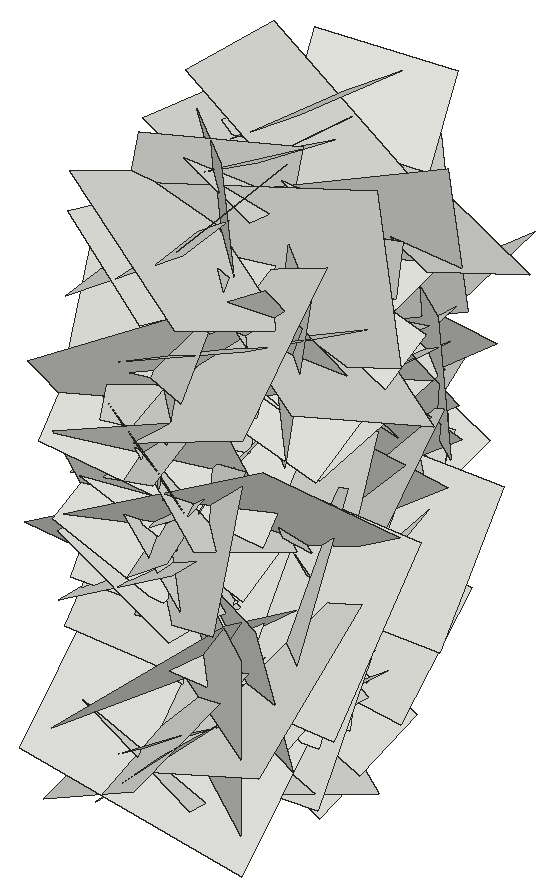
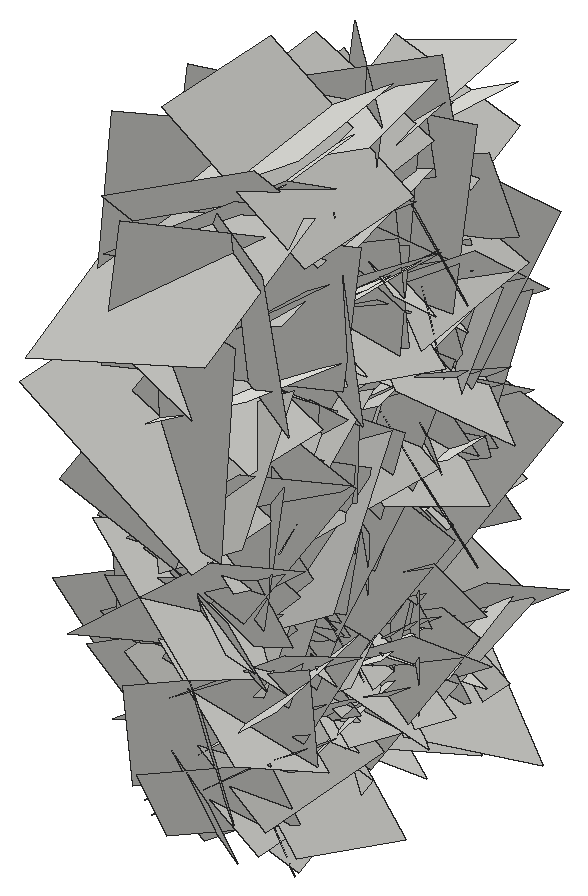
# SketchUp Ruby script. Lengths in inches.
U = 1.inch
M = Sketchup.active_model
def pt(a) = Geom::Point3d.new(a.map { |v| v * U })
def face(e, loops, mat)
  f = e.add_face(loops[0].map { |a| pt(a) })
  loops[1..].each { |l| e.add_face(l.map { |a| pt(a) }).erase! }
  f.material = f.back_material = mat if mat
  f
end
# faces: each face lists its corners as indices into pts; further lists are holes
def faces(e, pts, list, mat = nil) = list.each { |f| face(e, (f[0].is_a?(Array) ? f : [f]).map { |l| l.map { |i| pts[i] } }, mat) }
# xy, xz, yz: faces in a plane at the given z, y or x. An outline is a flat list of corners, or four numbers for a rectangle; further outlines are holes
def ring(l) = l.size == 4 ? [[l[0], l[1]], [l[2], l[1]], [l[2], l[3]], [l[0], l[3]]] : l.each_slice(2).to_a
def flat(e, list, mat, &to3) = list.each { |f| face(e, (f[0].is_a?(Array) ? f : [f]).map { |l| ring(l).map { |u, v| to3.(u, v) } }, mat) }
def xy(e, z, list, mat = nil) = flat(e, list, mat) { |x, y| [x, y, z] }
def xz(e, y, list, mat = nil) = flat(e, list, mat) { |x, z| [x, y, z] }
def yz(e, x, list, mat = nil) = flat(e, list, mat) { |y, z| [x, y, z] }
def lines(e, pts, list) = list.each { |a, b| e.add_line(pt(pts[a]), pt(pts[b])) }
# prism: a flat outline (further loops are holes) pulled along v
def prism(e, loops, v, mat = nil)
  f = face(e, loops, mat); d = Geom::Vector3d.new(v.map { |x| x * U })
  f.pushpull(f.normal.samedirection?(d) ? d.length : -d.length)
end
def box(e, o, s, mat = nil) = prism(e, [[o, [o[0] + s[0], o[1], o[2]], [o[0] + s[0], o[1] + s[1], o[2]], [o[0], o[1] + s[1], o[2]]]], [0, 0, s[2]], mat)
def at(x, y, z, deg = 0) = Geom::Transformation.translation(pt([x, y, z])) * Geom::Transformation.rotation(ORIGIN, Z_AXIS, deg.degrees)
def axes(o, x, y, z) = Geom::Transformation.new([*x, 0, *y, 0, *z, 0, *pt(o).to_a, 1])
def part(name) = M.definitions.add(name)
# library, detail: a bought-in or finely detailed component or shape, given as its bounding box
def library(name, o, s) = part(name).tap { |d| box(d.entities, o, s) }
def detail(e, o, s) = box(e.add_group.entities, o, s)
def put(e, d, t, mat = nil) = e.add_instance(d, t).tap { |i| i.material = mat if mat }
def group(e, t, mat = nil) = e.add_group.tap { |g| g.transformation = t; g.material = mat if mat }.entities
root = M.entities
c1 = part("Component\#6")
p = [[0.01,0,0],[0,3.24,4.54],[4.32,3.24,4.54],[4.33,0,0]]
faces(c1.entities,p,[[0,1,2,3]])
put(root,c1,axes([34.14,144.73,33.27],[-0.16555,-0.76551,-0.15352],[0.02389,-0.16091,0.77946],[0.82725,-0.14855,-0.05323]))
put(root,c1,axes([34.14,146.45,21.25],[-0.00375,0.2874,0.54008],[0.0654,0.5375,-0.28562],[0.64519,-0.05282,0.03209]))
put(root,c1,axes([34.14,136.92,29.78],[0.03864,0.57092,0.32429],[-0.05823,0.3263,-0.56829],[0.69355,-0.00442,-0.06578]))
put(root,c1,axes([34.14,144.18,33.46],[-0.08879,-0.56105,-0.39599],[0.0694,-0.40364,0.55803],[0.72461,-0.03009,-0.10197]))
put(root,c1,axes([38.11,149.17,29.19],[-0.22051,-0.77582,-0.34275],[0.07369,-0.36732,0.78924],[-0.89602,0.16072,0.14925]))
put(root,c1,axes([34.14,141.16,33.73],[0.01034,-0.20439,-0.70125],[-0.11317,-0.69418,0.20085],[0.76594,-0.09981,0.03914]))
put(root,c1,axes([34.14,145.72,37.21],[0.0202,-0.65006,0.07365],[-0.02062,0.07308,0.65011],[0.69316,0.02112,0.01719]))
put(root,c1,axes([34.14,146.3,23.53],[-0.0913,-0.50535,0.50896],[0.05568,0.5068,0.51209],[0.75823,-0.09807,0.02368]))
put(root,c1,axes([34.14,145.7,22.51],[-0.08358,0.19729,0.79599],[-0.0899,0.79341,-0.20506],[0.86462,0.10156,0.05562]))
put(root,c1,axes([38.11,145.12,23.07],[0.0526,-0.82286,-0.58821],[-0.0059,-0.58914,0.82367],[-1.07215,-0.03713,-0.03339]))
put(root,c1,axes([34.14,147.44,21.48],[0.11936,-0.32986,-0.48912],[-0.02265,-0.49991,0.33221],[0.62494,0.04489,0.10546]))
put(root,c1,axes([38.11,137.68,27.62],[-0.00267,0.49736,0.77514],[-0.05686,0.77375,-0.49665],[-0.97459,-0.04651,0.02685]))
put(root,c1,axes([38.11,136.3,32.46],[0.17238,0.91042,0.71253],[0.07022,0.71102,-0.92361],[-1.22345,0.16908,0.04738]))
put(root,c1,axes([34.14,137.77,24.11],[-0.1419,0.78136,-0.16109],[0.04598,-0.15597,-0.79258],[0.84441,0.13979,0.01609]))
put(root,c1,axes([34.14,143.53,22.21],[-0.15224,-0.84766,-0.36991],[-0.10957,-0.35729,0.85887],[0.97421,-0.17265,0.03879]))
put(root,c1,axes([38.11,135.48,23.28],[0.21581,1.04519,0.5846],[0.09636,0.57779,-1.06467],[-1.26577,0.22219,0.01862]))
put(root,c1,axes([34.14,145.6,27.28],[0.00806,0.29423,-0.56577],[0.12293,-0.55701,-0.28812],[0.6647,0.09945,0.06014]))
put(root,c1,axes([38.11,141.63,23.18],[0.01995,1.00092,0.30572],[0.13829,0.30114,-0.99396],[-1.10071,0.05598,-0.11933]))
put(root,c1,axes([38.11,145.42,24.52],[0.2647,-0.88765,0.75819],[0.01358,0.77738,0.90589],[-1.23735,-0.18136,0.17214]))
put(root,c1,axes([34.14,144.6,22.65],[-0.17478,-0.82558,-0.09028],[0.09417,-0.10904,0.83495],[0.87528,-0.15312,-0.10786]))
put(root,c1,axes([38.11,142.67,41.25],[0.05619,0.9574,-0.08237],[-0.00834,-0.08206,-0.95886],[-1.01856,0.05349,0.00331]))
put(root,c1,axes([38.11,148.52,32.35],[-0.08011,-0.79067,-0.06214],[-0.07476,-0.05548,0.79163],[-0.83736,0.0806,-0.06473]))
put(root,c1,axes([34.14,140.84,40.56],[-0.05261,0.712,-0.12967],[0.10362,-0.12219,-0.70833],[0.7601,0.06594,0.08758]))
put(root,c1,axes([34.14,143.38,25.93],[-0.00088,-0.66729,0.07011],[0.1194,0.06898,0.65784],[0.70113,-0.01259,-0.11194]))
put(root,c1,axes([34.14,144.05,31.85],[-0.11078,0.17753,-0.74918],[0.12323,-0.74375,-0.19246],[0.80677,0.13798,-0.07348]))
put(root,c1,axes([38.11,138.53,29.67],[-0.03677,-0.4198,0.69058],[-0.10131,0.68849,0.41374],[-0.85065,-0.06385,-0.07912]))
put(root,c1,axes([38.11,150.98,27.43],[-0.11329,-0.77541,-0.3635],[0.07754,-0.37325,0.77469],[-0.90445,0.06513,0.11195]))
put(root,c1,axes([38.11,149.13,24.11],[0.03147,-0.85153,-0.39996],[0.02133,-0.3995,0.85202],[-0.997,-0.03542,0.00561]))
put(root,c1,axes([38.11,144.71,33.13],[0.16995,0.04512,1.05289],[0.00982,1.0649,-0.04705],[-1.11704,0.01623,0.15977]))
put(root,c1,axes([34.14,143.64,28.51],[0.01569,-0.00258,-0.72773],[0.02057,-0.72762,0.00297],[0.77112,0.01947,0.01473]))
put(root,c1,axes([38.11,137.85,30.84],[0.06669,0.91948,0.38333],[0.06841,0.37952,-0.92095],[-1.05374,0.08283,-0.03553]))
put(root,c1,axes([38.11,147.08,31.53],[0.0186,0.21399,-0.90436],[0.04027,-0.90393,-0.21315],[-0.98427,-0.03294,-0.02581]))
put(root,c1,axes([34.14,144.98,23.12],[0.11015,0.70988,0.06167],[-0.04855,0.06885,-0.71532],[0.75374,-0.09931,-0.05509]))
put(root,c1,axes([34.14,140.76,35.5625],[0.0095,0.80566,-0.00603],[-0.04784,-0.00552,-0.80445],[0.85268,-0.00929,-0.04507]))
put(root,c1,axes([34.14,146.7,34.04],[-0.22474,0.77203,-0.6543],[-0.03576,-0.67353,-0.78378],[1.07212,0.13937,-0.1633]))
put(root,c1,axes([38.11,141.61,27.46],[0.15544,0.8369,-0.58263],[0.03072,-0.5918,-0.84279],[-1.08048,0.10358,-0.10778]))
put(root,c1,axes([38.11,145.6875,25.3],[0.21495,-0.77208,-0.77151],[0.06755,-0.77499,0.79232],[-1.15499,-0.18901,-0.09724]))
put(root,c1,axes([38.11,147.86,21.63],[0.08807,-1.00346,0.13322],[0.11481,0.14172,0.99989],[-1.06685,-0.06759,0.1186]))
put(root,c1,axes([34.14,139.84,37.375],[0.13047,0.02824,0.77],[-0.11824,0.77221,-0.01049],[0.80815,0.10842,-0.12584]))
put(root,c1,axes([38.11,144.76,23.61],[-0.10873,-0.7568,0.02149],[0.01122,0.02025,0.76368],[-0.80245,0.10283,0.00777]))
put(root,c1,axes([34.14,149.44,28.46],[-0.01637,-0.35652,-0.61871],[0.18604,-0.60176,0.34238],[0.7337,0.14463,-0.10062]))
put(root,c1,axes([34.14,137.14,29.31],[0.00249,0.75761,-0.01469],[0.08098,-0.01485,-0.75375],[0.79913,-0.00085,0.07643]))
put(root,c1,axes([34.14,137.53,34.5],[-0.08019,0.3809,0.76753],[0.04804,0.77121,-0.37826],[0.90698,-0.00717,0.08789]))
put(root,c1,axes([38.11,139.47,36.72],[-0.15825,-0.66033,0.08813],[-0.02764,0.09604,0.67542],[-0.70562,0.14433,-0.04622]))
put(root,c1,axes([34.14,139.47,36.72],[0.15825,-0.66033,0.08813],[0.02764,0.09604,0.67542],[0.70562,0.14433,-0.04622]))
put(root,c1,axes([38.11,137.53,34.5],[0.08019,0.3809,0.76753],[-0.04804,0.77121,-0.37826],[-0.90698,-0.00717,0.08789]))
put(root,c1,axes([38.11,137.14,29.31],[-0.00249,0.75761,-0.01469],[-0.08098,-0.01485,-0.75375],[-0.79913,-0.00085,0.07643]))
put(root,c1,axes([38.11,149.44,28.46],[0.01637,-0.35652,-0.61871],[-0.18604,-0.60176,0.34238],[-0.7337,0.14463,-0.10062]))
put(root,c1,axes([34.14,144.76,23.61],[0.10873,-0.7568,0.02149],[-0.01122,0.02025,0.76368],[0.80245,0.10283,0.00777]))
put(root,c1,axes([38.11,139.84,37.375],[-0.13047,0.02824,0.77],[0.11824,0.77221,-0.01049],[-0.80815,0.10842,-0.12584]))
put(root,c1,axes([34.14,147.86,21.63],[-0.08807,-1.00346,0.13322],[-0.11481,0.14172,0.99989],[1.06685,-0.06759,0.1186]))
put(root,c1,axes([34.14,145.6875,25.3],[-0.21495,-0.77208,-0.77151],[-0.06755,-0.77499,0.79232],[1.15499,-0.18901,-0.09724]))
put(root,c1,axes([34.14,141.61,27.46],[-0.15544,0.8369,-0.58263],[-0.03072,-0.5918,-0.84279],[1.08048,0.10358,-0.10778]))
put(root,c1,axes([38.11,146.7,34.04],[0.22474,0.77203,-0.6543],[0.03576,-0.67353,-0.78378],[-1.07212,0.13937,-0.1633]))
put(root,c1,axes([38.11,140.76,35.5625],[-0.0095,0.80566,-0.00603],[0.04784,-0.00552,-0.80445],[-0.85268,-0.00929,-0.04507]))
put(root,c1,axes([38.11,144.98,23.12],[-0.11015,0.70988,0.06167],[0.04855,0.06885,-0.71532],[-0.75374,-0.09931,-0.05509]))
put(root,c1,axes([34.14,147.08,31.53],[-0.0186,0.21399,-0.90436],[-0.04027,-0.90393,-0.21315],[0.98427,-0.03294,-0.02581]))
put(root,c1,axes([34.14,137.85,30.84],[-0.06669,0.91948,0.38333],[-0.06841,0.37952,-0.92095],[1.05374,0.08283,-0.03553]))
put(root,c1,axes([38.11,143.64,28.51],[-0.01569,-0.00258,-0.72773],[-0.02057,-0.72762,0.00297],[-0.77112,0.01947,0.01473]))
put(root,c1,axes([34.14,144.71,33.13],[-0.16995,0.04512,1.05289],[-0.00982,1.0649,-0.04705],[1.11704,0.01623,0.15977]))
put(root,c1,axes([34.14,149.13,24.11],[-0.03147,-0.85153,-0.39996],[-0.02133,-0.3995,0.85202],[0.997,-0.03542,0.00561]))
put(root,c1,axes([34.14,150.98,27.43],[0.11329,-0.77541,-0.3635],[-0.07754,-0.37325,0.77469],[0.90445,0.06513,0.11195]))
put(root,c1,axes([34.14,138.53,29.67],[0.03677,-0.4198,0.69058],[0.10131,0.68849,0.41374],[0.85065,-0.06385,-0.07912]))
put(root,c1,axes([38.11,144.05,31.85],[0.11078,0.17753,-0.74918],[-0.12323,-0.74375,-0.19246],[-0.80677,0.13798,-0.07348]))
put(root,c1,axes([38.11,143.38,25.93],[0.00088,-0.66729,0.07011],[-0.1194,0.06898,0.65784],[-0.70113,-0.01259,-0.11194]))
put(root,c1,axes([38.11,140.84,40.56],[0.05261,0.712,-0.12967],[-0.10362,-0.12219,-0.70833],[-0.7601,0.06594,0.08758]))
put(root,c1,axes([34.14,148.52,32.35],[0.08011,-0.79067,-0.06214],[0.07476,-0.05548,0.79163],[0.83736,0.0806,-0.06473]))
put(root,c1,axes([34.14,142.67,41.25],[-0.05619,0.9574,-0.08237],[0.00834,-0.08206,-0.95886],[1.01856,0.05349,0.00331]))
put(root,c1,axes([38.11,144.6,22.65],[0.17478,-0.82558,-0.09028],[-0.09417,-0.10904,0.83495],[-0.87528,-0.15312,-0.10786]))
put(root,c1,axes([34.14,145.42,24.52],[-0.2647,-0.88765,0.75819],[-0.01358,0.77738,0.90589],[1.23735,-0.18136,0.17214]))
put(root,c1,axes([34.14,141.63,23.18],[-0.01995,1.00092,0.30572],[-0.13829,0.30114,-0.99396],[1.10071,0.05598,-0.11933]))
put(root,c1,axes([38.11,145.6,27.28],[-0.00806,0.29423,-0.56577],[-0.12293,-0.55701,-0.28812],[-0.6647,0.09945,0.06014]))
put(root,c1,axes([34.14,135.48,23.28],[-0.21581,1.04519,0.5846],[-0.09636,0.57779,-1.06467],[1.26577,0.22219,0.01862]))
put(root,c1,axes([38.11,143.53,22.21],[0.15224,-0.84766,-0.36991],[0.10957,-0.35729,0.85887],[-0.97421,-0.17265,0.03879]))
put(root,c1,axes([38.11,137.77,24.11],[0.1419,0.78136,-0.16109],[-0.04598,-0.15597,-0.79258],[-0.84441,0.13979,0.01609]))
put(root,c1,axes([34.14,136.3,32.46],[-0.17238,0.91042,0.71253],[-0.07022,0.71102,-0.92361],[1.22345,0.16908,0.04738]))
put(root,c1,axes([34.14,137.68,27.62],[0.00267,0.49736,0.77514],[0.05686,0.77375,-0.49665],[0.97459,-0.04651,0.02685]))
put(root,c1,axes([38.11,147.44,21.48],[-0.11936,-0.32986,-0.48912],[0.02265,-0.49991,0.33221],[-0.62494,0.04489,0.10546]))
put(root,c1,axes([34.14,145.12,23.07],[-0.0526,-0.82286,-0.58821],[0.0059,-0.58914,0.82367],[1.07215,-0.03713,-0.03339]))
put(root,c1,axes([38.11,145.7,22.51],[0.08358,0.19729,0.79599],[0.0899,0.79341,-0.20506],[-0.86462,0.10156,0.05562]))
put(root,c1,axes([38.11,146.3,23.53],[0.0913,-0.50535,0.50896],[-0.05568,0.5068,0.51209],[-0.75823,-0.09807,0.02368]))
put(root,c1,axes([38.11,145.72,37.21],[-0.0202,-0.65006,0.07365],[0.02062,0.07308,0.65011],[-0.69316,0.02112,0.01719]))
put(root,c1,axes([38.11,141.16,33.73],[-0.01034,-0.20439,-0.70125],[0.11317,-0.69418,0.20085],[-0.76594,-0.09981,0.03914]))
put(root,c1,axes([34.14,149.17,29.19],[0.22051,-0.77582,-0.34275],[-0.07369,-0.36732,0.78924],[0.89602,0.16072,0.14925]))
put(root,c1,axes([38.11,144.18,33.46],[0.08879,-0.56105,-0.39599],[-0.0694,-0.40364,0.55803],[-0.72461,-0.03009,-0.10197]))
put(root,c1,axes([38.11,136.92,29.78],[-0.03864,0.57092,0.32429],[0.05823,0.3263,-0.56829],[-0.69355,-0.00442,-0.06578]))
put(root,c1,axes([38.11,146.45,21.25],[0.00375,0.2874,0.54008],[-0.0654,0.5375,-0.28562],[-0.64519,-0.05282,0.03209]))
put(root,c1,axes([38.11,144.73,33.27],[0.16555,-0.76551,-0.15352],[-0.02389,-0.16091,0.77946],[-0.82725,-0.14855,-0.05323]))
put(root,c1,axes([34.14,144.65,25.96],[0.15377,0.53431,0.65108],[0.06081,0.65286,-0.54856],[0.89071,-0.13681,-0.07495]))
put(root,c1,axes([38.11,139.71,39.61],[-0.08624,0.67106,-0.00672],[0.16105,0.01183,-0.6586],[-0.69289,-0.08077,-0.15225]))
put(root,c1,axes([34.14,143.41,32.67],[-0.00295,0.89075,-0.72818],[-0.15415,-0.72261,-0.88339],[1.20976,-0.08991,-0.11434]))
put(root,c1,axes([34.14,146.5,19.86],[0.14062,-0.87102,0.18651],[0.03259,0.19294,0.87915],[0.94365,0.12313,-0.05815]))
put(root,c1,axes([34.14,145.05,38.54],[-0.26561,0.06521,-1.32838],[-0.06869,-1.35074,-0.05408],[1.4081,-0.05359,-0.25321]))
put(root,c1,axes([34.14,142.58,23.75],[0.11698,0.88265,-0.34817],[-0.00423,-0.35009,-0.88876],[1.00576,-0.10414,0.03675]))
put(root,c1,axes([34.14,141.41,21.99],[0.04242,-1.10503,0.33762],[-0.18816,0.32793,1.09436],[1.21025,0.08972,0.15831]))
put(root,c1,axes([38.11,145.49,24.46],[0.14807,-0.32942,-0.64401],[-0.00647,-0.65643,0.33444],[-0.76675,-0.05808,-0.12719]))
put(root,c1,axes([34.14,138.75,33.42],[0.07987,0.93748,-0.3836],[-0.04246,-0.3816,-0.94046],[1.07286,-0.0849,-0.00867]))
put(root,c1,axes([38.11,142.8,24.59],[0.06246,-0.31977,0.5346],[-0.03506,0.53462,0.32343],[-0.65938,-0.05871,0.03344]))
put(root,c1,axes([38.11,142.28,27.34],[0.09885,-0.42767,0.49172],[-0.03253,0.4933,0.43487],[-0.69002,-0.08452,0.04994]))
put(root,c1,axes([34.14,139.49,21.74],[0.04906,0.46783,0.90513],[0.0041,0.90598,-0.46846],[1.08001,-0.02469,-0.03934]))
put(root,c1,axes([38.11,149.12,29.1],[0.10824,-0.19319,-0.65872],[0.02698,-0.66445,0.19881],[-0.72715,-0.05341,-0.09068]))
put(root,c1,axes([34.14,145.04,25.97],[-0.0145,-0.85349,0.83598],[-0.13626,0.83223,0.84756],[1.25903,0.08024,0.10136]))
put(root,c1,axes([38.11,141.05,35.76],[0.06877,-0.60814,0.14272],[0.00885,0.14432,0.61116],[-0.66208,-0.06124,0.02299]))
put(root,c1,axes([38.11,149.56,39.6],[0.17317,-0.50739,-0.45031],[-0.03865,-0.46908,0.51531],[-0.71806,-0.09712,-0.13634]))
put(root,c1,axes([38.11,140.39,26.94],[0.03872,-0.62994,0.14227],[0.11345,0.14643,0.62088],[-0.67508,-0.01152,0.1125]))
put(root,c1,axes([38.11,144.97,35.07],[0.07722,-0.5315,-0.34657],[0.05738,-0.34237,0.53643],[-0.67013,-0.09056,0.006]))
put(root,c1,axes([34.14,139.67,30.68],[-0.09112,-0.77438,0.96294],[-0.03313,0.96632,0.77431],[1.3094,-0.02944,0.0866]))
put(root,c1,axes([34.14,138.43,27.8],[0.10648,0.28124,1.16655],[-0.16097,1.1642,-0.2676],[1.26174,0.12479,-0.13259]))
put(root,c1,axes([34.14,140.69,35.43],[0.02714,1.22478,0.26938],[-0.1382,0.27058,-1.21783],[1.3221,0.00314,-0.13283]))
put(root,c1,axes([34.14,137.65,40.3125],[0.15365,0.92766,-0.3555],[0.07441,-0.36793,-0.93147],[1.05042,-0.10963,0.11798]))
put(root,c1,axes([38.11,136.62,23.89],[0.08859,0.63974,0.04756],[0.12242,0.03217,-0.63572],[-0.66888,0.09062,-0.11005]))
put(root,c1,axes([34.14,149.09,36.34],[-0.1737,0.35213,-1.24285],[0.08,-1.24806,-0.36356],[1.36694,0.11779,-0.13666]))
put(root,c1,axes([34.14,146.73,29.36],[-0.09029,-1.26195,0.03468],[0.03892,0.03227,1.26436],[1.33761,-0.08612,-0.03444]))
put(root,c1,axes([34.14,141.99,33.2],[0.15631,-0.03731,1.01998],[0.08418,1.02787,0.02612],[1.07863,-0.07482,-0.14985]))
put(root,c1,axes([34.14,141.2,30.22],[0.14348,-0.5033,-0.91823],[0.06175,-0.92081,0.51331],[1.10823,0.11647,0.09028]))
put(root,c1,axes([34.14,143.42,27.33],[0.08667,-0.86973,1.01008],[-0.23887,0.9884,0.86929],[1.39256,0.22367,0.08625]))
put(root,c1,axes([34.14,142.6875,32.73],[-0.11413,-1.14483,0.29443],[0.2702,0.26621,1.12831],[1.22353,-0.16558,-0.2217]))
put(root,c1,axes([34.14,143.97,23.32],[0.18437,0.48358,0.83906],[0.16998,0.82633,-0.50949],[1.01237,-0.22682,-0.06726]))
put(root,c1,axes([34.14,144,25.2],[0.04504,0.58566,0.95802],[0.11757,0.95183,-0.5868],[1.18441,-0.11675,0.02182]))
put(root,c1,axes([34.14,150.86,30.47],[0.14962,-1.13409,-0.09371],[-0.03493,-0.09847,1.14197],[1.20573,0.13788,0.04471]))
put(root,c1,axes([34.14,141.59,27.99],[-0.06396,0.08339,-1.32201],[-0.02487,-1.32324,-0.0824],[1.4039,-0.01964,-0.06169]))
put(root,c1,axes([34.14,145.76,27.48],[0.11303,-0.66031,-0.96553],[-0.02355,-0.9705,0.66125],[1.23968,0.04176,0.1006]))
put(root,c1,axes([34.14,149.48,27.53],[0.05839,-0.93868,-0.8352],[-0.07486,-0.83699,0.93604],[1.32974,-0.0059,0.08937]))
put(root,c1,axes([34.14,141.72,37.36],[0.19445,0.97106,0.50245],[-0.00165,0.50971,-0.98451],[1.15895,-0.1622,-0.0857]))
put(root,c1,axes([34.14,141.71,25.57],[-0.24627,-1.07768,0.84944],[0.21085,0.82598,1.10232],[1.43917,-0.30542,-0.01615]))
put(root,c1,axes([34.14,141.15,27.9],[0.10356,0.25866,-1.08582],[0.18317,-1.08033,-0.24181],[1.16891,0.14638,0.13409]))
put(root,c1,axes([34.14,145.83,38.68],[-0.04371,1.09164,-0.51046],[0.28885,-0.48908,-1.06793],[1.24431,0.15188,0.22998]))
put(root,c1,axes([34.14,140.25,33.3],[-0.10371,-0.10781,1.29757],[0.22808,1.282,0.12274],[1.36119,-0.22303,0.07829]))
put(root,c1,axes([34.14,139.39,34.34],[0.15089,0.92592,0.71699],[0.08883,0.71236,-0.93659],[1.23815,-0.16395,-0.02018]))
put(root,c1,axes([34.14,142.42,32.89],[0.18672,-0.42722,1.28431],[-0.1337,1.28432,0.44452],[1.42847,0.17605,-0.12627]))
put(root,c1,axes([34.14,142.63,35.02],[0.11092,-0.98462,-0.77371],[0.1183,-0.76598,0.98988],[1.32209,0.15114,-0.02366]))
put(root,c1,axes([34.14,137.42,26.21],[0.14568,0.69276,1.17725],[0.03045,1.18146,-0.69859],[1.44759,-0.09457,-0.10377]))
put(root,c1,axes([34.14,143.09,24.72],[0.05768,-1.1082,-0.74759],[0.23067,-0.73089,1.09928],[1.3981,0.16631,-0.15052]))
put(root,c1,axes([34.14,141,38.04],[0.14868,1.2474,-0.57055],[0.09146,-0.58042,-1.24775],[1.45112,-0.09122,0.1371]))
